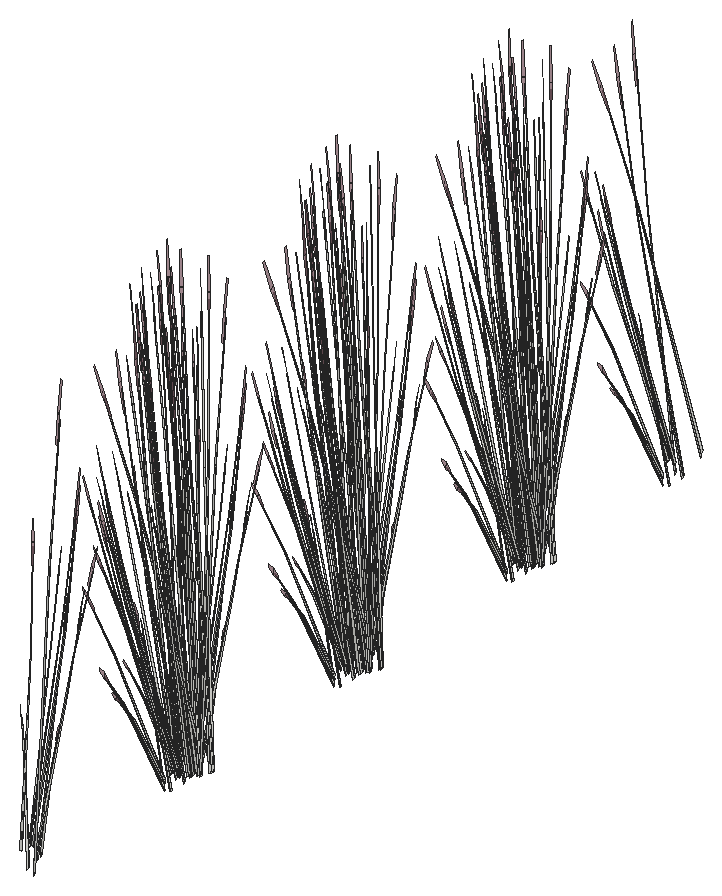
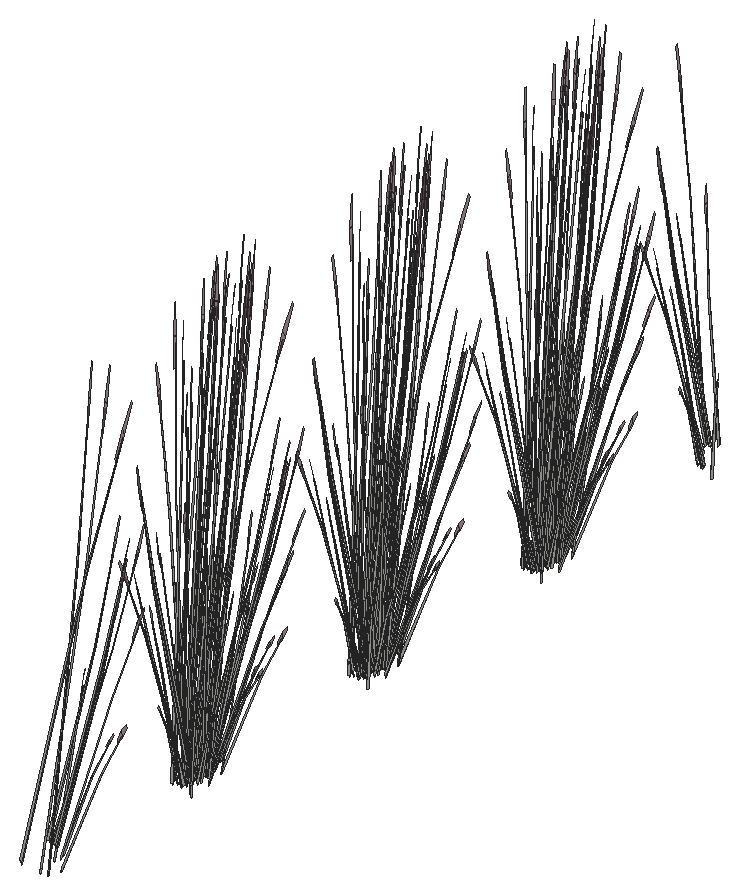
# SketchUp Ruby script. Lengths in inches.
U = 1.inch
M = Sketchup.active_model
def pt(a) = Geom::Point3d.new(a.map { |v| v * U })
def face(e, loops, mat)
  f = e.add_face(loops[0].map { |a| pt(a) })
  loops[1..].each { |l| e.add_face(l.map { |a| pt(a) }).erase! }
  f.material = f.back_material = mat if mat
  f
end
# faces: each face lists its corners as indices into pts; further lists are holes
def faces(e, pts, list, mat = nil) = list.each { |f| face(e, (f[0].is_a?(Array) ? f : [f]).map { |l| l.map { |i| pts[i] } }, mat) }
# xy, xz, yz: faces in a plane at the given z, y or x. An outline is a flat list of corners, or four numbers for a rectangle; further outlines are holes
def ring(l) = l.size == 4 ? [[l[0], l[1]], [l[2], l[1]], [l[2], l[3]], [l[0], l[3]]] : l.each_slice(2).to_a
def flat(e, list, mat, &to3) = list.each { |f| face(e, (f[0].is_a?(Array) ? f : [f]).map { |l| ring(l).map { |u, v| to3.(u, v) } }, mat) }
def xy(e, z, list, mat = nil) = flat(e, list, mat) { |x, y| [x, y, z] }
def xz(e, y, list, mat = nil) = flat(e, list, mat) { |x, z| [x, y, z] }
def yz(e, x, list, mat = nil) = flat(e, list, mat) { |y, z| [x, y, z] }
def lines(e, pts, list) = list.each { |a, b| e.add_line(pt(pts[a]), pt(pts[b])) }
# prism: a flat outline (further loops are holes) pulled along v
def prism(e, loops, v, mat = nil)
  f = face(e, loops, mat); d = Geom::Vector3d.new(v.map { |x| x * U })
  f.pushpull(f.normal.samedirection?(d) ? d.length : -d.length)
end
def box(e, o, s, mat = nil) = prism(e, [[o, [o[0] + s[0], o[1], o[2]], [o[0] + s[0], o[1] + s[1], o[2]], [o[0], o[1] + s[1], o[2]]]], [0, 0, s[2]], mat)
def at(x, y, z, deg = 0) = Geom::Transformation.translation(pt([x, y, z])) * Geom::Transformation.rotation(ORIGIN, Z_AXIS, deg.degrees)
def axes(o, x, y, z) = Geom::Transformation.new([*x, 0, *y, 0, *z, 0, *pt(o).to_a, 1])
def part(name) = M.definitions.add(name)
# library, detail: a bought-in or finely detailed component or shape, given as its bounding box
def library(name, o, s) = part(name).tap { |d| box(d.entities, o, s) }
def detail(e, o, s) = box(e.add_group.entities, o, s)
def put(e, d, t, mat = nil) = e.add_instance(d, t).tap { |i| i.material = mat if mat }
def group(e, t, mat = nil) = e.add_group.tap { |g| g.transformation = t; g.material = mat if mat }.entities
root = M.entities
M.materials.add("LightPink_Translucent").color = [144, 107, 117]
M.materials["LightPink_Translucent"].alpha = 0.75
c1 = part("blade")
p = [[2.15,0.21,22],[0,0.17,0],[0.09,0.45,0],[2.18,0.31,22],[2.29,0.31,22],[0.38,0.45,0],
  [2.48,0.24,33],[2.49,0.24,33],[2.48,0.22,33]]
faces(c1.entities,p,[[0,1,2,3],[4,5,2,3],[6,3,4,7],[8,0,3,6]])
c2 = part("seeds")
p = [[0.3,-0.1,1.38],[-0.01,-0.03,1.59],[-0.01,-0.03,0.03],[0.14,-0.07,-0.07],[0.29,-0.03,3],[0.15,0.01,3.11]]
faces(c2.entities,p,[[0,1,2,3],[1,0,4,5]],"LightPink_Translucent")
c3 = part("blade with seeds")
put(c3.entities,c1,at(0,0,0))
put(c3.entities,c2,axes([2.4,0.25,30.99],[1.5799,-0.05474,1.17369],[-0.12525,1.92788,0.29478],[-0.07173,-0.02425,1.56792]))
put(root,c3,axes([431.05,69.35,2.03],[0.09666,0.50384,-0.43945],[-0.36608,0.08814,-0.34039],[-0.10491,0.13533,0.84085]))
put(root,c3,axes([433.2,68.33,0.44],[-0.01028,-0.51954,1.21494],[0.46521,0.13467,0.51441],[-0.11003,0.28429,1.14681]))
put(root,c3,axes([430.6,70.64,-0.72],[0.05047,0.05513,1.51654],[0.08558,0.51079,-0.23168],[-0.11187,0.10892,0.25832]))
put(root,c3,axes([431.36,70.35,1.89],[-0.2546,0.29052,-0.30456],[-0.24101,-0.33173,0.39319],[-0.03667,0.16855,0.75234]))
put(root,c3,axes([431.52,71.47,0.38],[-0.00974,-0.3281,0.9878],[0.24334,0.23402,0.72577],[-0.04786,0.15639,0.21757]))
put(root,c3,axes([431.61,70.21,2.3],[0.26937,0.37076,-0.48779],[-0.28456,0.3247,-0.37783],[-0.04099,0.18838,0.93334]))
put(root,c3,axes([431.32,70.76,0.43],[0.34184,-0.09771,0.05596],[0.07859,0.39367,-0.74222],[-0.02167,0.19928,0.6653]))
put(root,c3,axes([431.53,70.04,2.59],[-0.00979,0.51041,-0.6782],[-0.4123,-0.03428,0.08184],[-0.04351,0.21623,0.95938]))
put(root,c3,axes([431.24,71.18,0.23],[0.11874,-0.08705,1.22981],[0.29317,0.26247,-0.26449],[-0.08726,0.22711,0.52581]))
put(root,c3,axes([431.39,70.76,0.89],[0.00827,-0.28486,1.32737],[0.37184,0.15046,0.18343],[-0.03222,0.30359,0.62678]))
put(root,c3,axes([432.74,89.46,2.28],[-0.17959,-0.44867,-0.61099],[0.36969,-0.25004,0.07373],[-0.042,-0.21679,0.8643]))
put(root,c3,axes([431.57,88.86,0.23],[-0.02279,0.18051,1.22981],[-0.33311,0.15111,-0.26449],[-0.07787,-0.23331,0.52581]))
put(root,c3,axes([432.6,89.37,2.03],[-0.3699,-0.13833,-0.43945],[0.12679,-0.47426,-0.34039],[-0.03392,-0.19095,0.84085]))
put(root,c3,axes([431.45,88.57,0.38],[0.19628,0.19205,0.9878],[-0.28586,0.11545,0.72577],[-0.06116,-0.1476,0.21757]))
put(root,c3,axes([431.93,89.59,2.28],[-0.32086,-0.26671,-0.61099],[0.22803,-0.46737,0.07373],[-0.11625,-0.15925,0.8643]))
put(root,c3,axes([431.82,89.24,1.89],[-0.05812,-0.44446,-0.30456],[0.33222,-0.11736,0.39319],[-0.08923,-0.12737,0.75234]))
put(root,c3,axes([431.3,89.15,-0.72],[-0.03645,0.07269,1.51654],[-0.36835,0.15672,-0.23168],[-0.08898,-0.14257,0.25832]))
put(root,c3,axes([431.9,91.15,-0.2],[-0.15453,-0.56584,-0.60058],[0.44514,-0.20379,-0.15763],[-0.01708,-0.19161,1.32568]))
put(root,c3,axes([431.78,89.6,2.03],[-0.37131,0.13117,-0.43945],[-0.06495,-0.49674,-0.34039],[-0.09973,-0.14235,0.84085]))
put(root,c3,axes([432.36,88.85,-0.17],[-0.26003,0.31656,-0.03348],[-0.23826,-0.3467,-0.15179],[-0.01677,-0.09824,0.50065]))
put(root,c3,axes([432.69,92.61,0.86],[0.32517,0.22251,1.30084],[-0.31856,0.47936,0.51441],[-0.14269,-0.28411,1.09053]))
put(root,c3,axes([430.99,91.07,-0.26],[0,-0.5518,-0.427],[0.42099,0,0],[0,-0.12568,1.35453]))
put(root,c3,axes([431.05,90.02,1.89],[-0.2141,-0.34548,-0.30456],[0.24447,-0.32704,0.39319],[-0.12421,-0.04976,0.75234]))
put(root,c3,axes([431.17,91.08,-0.26],[0.26266,-0.34428,-0.26641],[0.26266,0.34428,0.26641],[0,-0.11089,1.19518]))
put(root,c3,axes([431.07,89.43,-0.17],[-0.10855,0.45057,-0.03348],[-0.33409,-0.1386,-0.15179],[-0.05073,-0.0737,0.50065]))
put(root,c3,axes([432.09,91.71,0.29],[-0.42377,-0.26329,-0.25022],[0.20405,-0.55571,-0.43002],[-0.01332,-0.13644,1.37348]))
put(root,c3,axes([430.89,91.49,0.04],[-0.47052,0,0],[0,-0.61671,-0.44382],[0,-0.14046,1.40792]))
put(root,c3,axes([430.97,90.38,0.23],[0.07347,0.15363,1.22981],[-0.16929,0.41759,-0.26449],[-0.17383,-0.09981,0.52581]))
put(root,c3,axes([431.27,90.25,2.28],[-0.37615,-0.01329,-0.61099],[0.02526,-0.55946,0.07373],[-0.15935,-0.05904,0.8643]))
put(root,c3,axes([431.25,91.32,0],[-0.35001,0.46392,0.2645],[-0.35022,-0.45904,-0.31383],[-0.01222,-0.13174,1.41801]))
put(root,c3,axes([432.2,92.29,0.1],[0.09973,-0.65385,-0.20149],[0.47288,0.11397,0.44093],[-0.08263,-0.0903,1.34539]))
put(root,c3,axes([431.15,90.36,2.03],[-0.27323,0.36552,-0.43945],[-0.23929,-0.38612,-0.34039],[-0.13882,-0.05561,0.84085]))
put(root,c3,axes([430.53,90.85,0.38],[0.24023,-0.03948,0.9878],[-0.15239,0.3479,0.72577],[-0.11872,-0.05219,0.21757]))
put(root,c3,axes([431.17,91.58,0.13],[0,0.5518,0.427],[-0.42099,0,0],[0,-0.12568,1.35453]))
put(root,c3,axes([432.17,92.03,-0.1],[-0.22605,-0.46315,-0.38476],[0.34239,-0.32614,0.18517],[-0.07315,-0.05731,1.23533]))
put(root,c3,axes([432.13,91.86,0.34],[-0.18257,0.49721,0.38476],[-0.37935,-0.23929,-0.18517],[0,-0.11462,1.23533]))
put(root,c3,axes([431.97,92.2,-0.23],[-0.39143,-0.09047,-0.53624],[0.0826,-0.55804,-0.14074],[-0.11681,-0.06762,1.18365]))
put(root,c3,axes([432.26,91.98,0.03],[0.4756,0.11626,0.39349],[-0.09679,0.6566,0.15441],[-0.0695,-0.0634,1.36617]))
put(root,c3,axes([430.71,91.41,-0.72],[0.00954,0.08696,1.51654],[-0.19238,0.45414,-0.23168],[-0.13665,-0.02289,0.25832]))
put(root,c3,axes([431.55,93.05,-0.26],[-0.08839,-0.48081,-0.26641],[0.35106,-0.13653,0.26641],[-0.07077,-0.05545,1.19518]))
put(root,c3,axes([431.45,93.26,-0.26],[-0.35217,-0.2759,-0.427],[0.2105,-0.49473,0],[-0.08021,-0.06284,1.35453]))
put(root,c3,axes([430.67,91.22,1.89],[-0.31272,-0.15393,-0.30456],[0.09121,-0.44909,0.39319],[-0.1259,0.04118,0.75234]))
put(root,c3,axes([432.41,92.29,0.29],[-0.37992,0.36634,-0.25022],[-0.25264,-0.51764,-0.43002],[-0.09374,-0.05257,1.37348]))
put(root,c3,axes([432.375,92.45,0.25],[-0.07259,0.49245,0.12452],[-0.35466,-0.08548,-0.35559],[-0.06454,-0.05057,1.09]))
put(root,c3,axes([431.62,91.14,0.875],[0.10696,-0.07982,1.52275],[0.03688,0.55733,0.11917],[-0.23167,0.07395,0.54424]))
put(root,c3,axes([432.84,92.45,0.12],[-0.36743,-0.44413,-0.21665],[0.30918,-0.49872,0.47412],[-0.09894,0.05195,1.44665]))
put(root,c3,axes([431.87,93.3,0.13],[0.35217,0.2759,0.427],[-0.2105,0.49473,0],[-0.08021,-0.06284,1.35453]))
put(root,c3,axes([430.88,91.45,2.03],[-0.10194,0.50193,-0.43945],[-0.34951,-0.17204,-0.34039],[-0.14072,0.04602,0.84085]))
put(root,c3,axes([431.67,93.59,0.04],[-0.23526,0.55293,0],[-0.3936,-0.30836,-0.44382],[-0.08964,-0.07023,1.40792]))
put(root,c3,axes([432.65,92.36,-0.1],[-0.40861,0.03406,-0.38476],[-0.03695,-0.56543,0.18517],[-0.07315,0.05731,1.23533]))
put(root,c3,axes([433.1,93.67,-0.11],[-0.23233,-0.55486,-0.04422],[0.3936,-0.30836,0.44382],[-0.09699,0.05283,1.40722]))
put(root,c3,axes([433,93.6,-0.26],[-0.35106,-0.13653,-0.26641],[0.08839,-0.48081,0.26641],[-0.07077,0.05545,1.19518]))
put(root,c3,axes([430.46,92.625,0.23],[0.13077,0.0453,1.22981],[0.08428,0.46268,-0.26449],[-0.17763,0.08661,0.52581]))
put(root,c3,axes([430.19,93.59,0.38],[0.15682,-0.25009,0.9878],[0.06188,0.39591,0.72577],[-0.11333,0.07089,0.21757]))
put(root,c3,axes([432.9375,92.2,0.29],[0.04385,0.62963,-0.25022],[-0.45669,0.03807,-0.43002],[-0.08042,0.08387,1.37348]))
put(root,c3,axes([430.78,92.51,1.89],[-0.32754,0.07886,-0.30456],[-0.08649,-0.45081,0.39319],[-0.09386,0.12109,0.75234]))
put(root,c3,axes([432.66,92.69,-0.23],[-0.25345,0.41475,-0.53624],[-0.31485,-0.37608,-0.14074],[-0.10156,0.10346,1.18365]))
put(root,c3,axes([433.08,93.82,-0.26],[-0.35217,0.2759,-0.427],[-0.2105,-0.49473,0],[-0.08021,0.06284,1.35453]))
put(root,c3,axes([431.05,92.5625,2.03],[0.09666,0.50384,-0.43945],[-0.36608,0.08814,-0.34039],[-0.10491,0.13533,0.84085]))
put(root,c3,axes([433.2,91.54,0.44],[-0.01028,-0.51954,1.21494],[0.46521,0.13467,0.51441],[-0.11003,0.28429,1.14681]))
put(root,c3,axes([430.6,93.85,-0.72],[0.05047,0.05513,1.51654],[0.08558,0.51079,-0.23168],[-0.11187,0.10892,0.25832]))
put(root,c3,axes([431.36,93.56,1.89],[-0.2546,0.29052,-0.30456],[-0.24101,-0.33173,0.39319],[-0.03667,0.16855,0.75234]))
put(root,c3,axes([431.52,94.68,0.38],[-0.00974,-0.3281,0.9878],[0.24334,0.23402,0.72577],[-0.04786,0.15639,0.21757]))
put(root,c3,axes([431.61,93.42,2.3],[0.26937,0.37076,-0.48779],[-0.28456,0.3247,-0.37783],[-0.04099,0.18838,0.93334]))
put(root,c3,axes([431.32,93.97,0.43],[0.34184,-0.09771,0.05596],[0.07859,0.39367,-0.74222],[-0.02167,0.19928,0.6653]))
put(root,c3,axes([431.53,93.25,2.59],[-0.00979,0.51041,-0.6782],[-0.4123,-0.03428,0.08184],[-0.04351,0.21623,0.95938]))
put(root,c3,axes([431.24,94.39,0.23],[0.11874,-0.08705,1.22981],[0.29317,0.26247,-0.26449],[-0.08726,0.22711,0.52581]))
put(root,c3,axes([431.39,93.97,0.89],[0.00827,-0.28486,1.32737],[0.37184,0.15046,0.18343],[-0.03222,0.30359,0.62678]))
put(root,c3,axes([431.57,112.55,0.23],[-0.02279,0.18051,1.22981],[-0.33311,0.15111,-0.26449],[-0.07787,-0.23331,0.52581]))
put(root,c3,axes([432.6,113.06,2.03],[-0.3699,-0.13833,-0.43945],[0.12679,-0.47426,-0.34039],[-0.03392,-0.19095,0.84085]))
put(root,c3,axes([431.45,112.26,0.38],[0.19628,0.19205,0.9878],[-0.28586,0.11545,0.72577],[-0.06116,-0.1476,0.21757]))
put(root,c3,axes([431.93,113.28,2.28],[-0.32086,-0.26671,-0.61099],[0.22803,-0.46737,0.07373],[-0.11625,-0.15925,0.8643]))
put(root,c3,axes([431.82,112.92,1.89],[-0.05812,-0.44446,-0.30456],[0.33222,-0.11736,0.39319],[-0.08923,-0.12737,0.75234]))
put(root,c3,axes([431.3,112.84,-0.72],[-0.03645,0.07269,1.51654],[-0.36835,0.15672,-0.23168],[-0.08898,-0.14257,0.25832]))
put(root,c3,axes([431.9,114.84,-0.2],[-0.15453,-0.56584,-0.60058],[0.44514,-0.20379,-0.15763],[-0.01708,-0.19161,1.32568]))
put(root,c3,axes([431.78,113.29,2.03],[-0.37131,0.13117,-0.43945],[-0.06495,-0.49674,-0.34039],[-0.09973,-0.14235,0.84085]))
put(root,c3,axes([432.36,112.54,-0.17],[-0.26003,0.31656,-0.03348],[-0.23826,-0.3467,-0.15179],[-0.01677,-0.09824,0.50065]))
put(root,c3,axes([432.69,116.29,0.86],[0.32517,0.22251,1.30084],[-0.31856,0.47936,0.51441],[-0.14269,-0.28411,1.09053]))
put(root,c3,axes([430.99,114.76,-0.26],[0,-0.5518,-0.427],[0.42099,0,0],[0,-0.12568,1.35453]))
put(root,c3,axes([431.05,113.71,1.89],[-0.2141,-0.34548,-0.30456],[0.24447,-0.32704,0.39319],[-0.12421,-0.04976,0.75234]))
put(root,c3,axes([431.17,114.77,-0.26],[0.26266,-0.34428,-0.26641],[0.26266,0.34428,0.26641],[0,-0.11089,1.19518]))
put(root,c3,axes([431.07,113.12,-0.17],[-0.10855,0.45057,-0.03348],[-0.33409,-0.1386,-0.15179],[-0.05073,-0.0737,0.50065]))
put(root,c3,axes([432.09,115.39,0.29],[-0.42377,-0.26329,-0.25022],[0.20405,-0.55571,-0.43002],[-0.01332,-0.13644,1.37348]))
put(root,c3,axes([430.89,115.17,0.04],[-0.47052,0,0],[0,-0.61671,-0.44382],[0,-0.14046,1.40792]))
put(root,c3,axes([430.97,114.07,0.23],[0.07347,0.15363,1.22981],[-0.16929,0.41759,-0.26449],[-0.17383,-0.09981,0.52581]))
put(root,c3,axes([431.27,113.9375,2.28],[-0.37615,-0.01329,-0.61099],[0.02526,-0.55946,0.07373],[-0.15935,-0.05904,0.8643]))
put(root,c3,axes([431.25,115.01,0],[-0.35001,0.46392,0.2645],[-0.35022,-0.45904,-0.31383],[-0.01222,-0.13174,1.41801]))
put(root,c3,axes([432.2,115.98,0.1],[0.09973,-0.65385,-0.20149],[0.47288,0.11397,0.44093],[-0.08263,-0.0903,1.34539]))
put(root,c3,axes([431.15,114.05,2.03],[-0.27323,0.36552,-0.43945],[-0.23929,-0.38612,-0.34039],[-0.13882,-0.05561,0.84085]))
put(root,c3,axes([430.53,114.53,0.38],[0.24023,-0.03948,0.9878],[-0.15239,0.3479,0.72577],[-0.11872,-0.05219,0.21757]))
put(root,c3,axes([431.17,115.27,0.13],[0,0.5518,0.427],[-0.42099,0,0],[0,-0.12568,1.35453]))
put(root,c3,axes([432.17,115.71,-0.1],[-0.22605,-0.46315,-0.38476],[0.34239,-0.32614,0.18517],[-0.07315,-0.05731,1.23533]))
put(root,c3,axes([432.13,115.55,0.34],[-0.18257,0.49721,0.38476],[-0.37935,-0.23929,-0.18517],[0,-0.11462,1.23533]))
put(root,c3,axes([431.97,115.89,-0.23],[-0.39143,-0.09047,-0.53624],[0.0826,-0.55804,-0.14074],[-0.11681,-0.06762,1.18365]))
put(root,c3,axes([432.26,115.66,0.03],[0.4756,0.11626,0.39349],[-0.09679,0.6566,0.15441],[-0.0695,-0.0634,1.36617]))
put(root,c3,axes([430.71,115.1,-0.72],[0.00954,0.08696,1.51654],[-0.19238,0.45414,-0.23168],[-0.13665,-0.02289,0.25832]))
put(root,c3,axes([431.55,116.74,-0.26],[-0.08839,-0.48081,-0.26641],[0.35106,-0.13653,0.26641],[-0.07077,-0.05545,1.19518]))
put(root,c3,axes([431.45,116.95,-0.26],[-0.35217,-0.2759,-0.427],[0.2105,-0.49473,0],[-0.08021,-0.06284,1.35453]))
put(root,c3,axes([430.67,114.91,1.89],[-0.31272,-0.15393,-0.30456],[0.09121,-0.44909,0.39319],[-0.1259,0.04118,0.75234]))
put(root,c3,axes([432.41,115.97,0.29],[-0.37992,0.36634,-0.25022],[-0.25264,-0.51764,-0.43002],[-0.09374,-0.05257,1.37348]))
put(root,c3,axes([432.375,116.13,0.25],[-0.07259,0.49245,0.12452],[-0.35466,-0.08548,-0.35559],[-0.06454,-0.05057,1.09]))
put(root,c3,axes([431.62,114.83,0.875],[0.10696,-0.07982,1.52275],[0.03688,0.55733,0.11917],[-0.23167,0.07395,0.54424]))
put(root,c3,axes([432.84,116.14,0.12],[-0.36743,-0.44413,-0.21665],[0.30918,-0.49872,0.47412],[-0.09894,0.05195,1.44665]))
put(root,c3,axes([431.87,116.99,0.13],[0.35217,0.2759,0.427],[-0.2105,0.49473,0],[-0.08021,-0.06284,1.35453]))
put(root,c3,axes([430.88,115.13,2.03],[-0.10194,0.50193,-0.43945],[-0.34951,-0.17204,-0.34039],[-0.14072,0.04602,0.84085]))
put(root,c3,axes([431.67,117.28,0.04],[-0.23526,0.55293,0],[-0.3936,-0.30836,-0.44382],[-0.08964,-0.07023,1.40792]))
put(root,c3,axes([432.65,116.05,-0.1],[-0.40861,0.03406,-0.38476],[-0.03695,-0.56543,0.18517],[-0.07315,0.05731,1.23533]))
put(root,c3,axes([433.1,117.36,-0.11],[-0.23233,-0.55486,-0.04422],[0.3936,-0.30836,0.44382],[-0.09699,0.05283,1.40722]))
put(root,c3,axes([433,117.29,-0.26],[-0.35106,-0.13653,-0.26641],[0.08839,-0.48081,0.26641],[-0.07077,0.05545,1.19518]))
put(root,c3,axes([430.46,116.3125,0.23],[0.13077,0.0453,1.22981],[0.08428,0.46268,-0.26449],[-0.17763,0.08661,0.52581]))
put(root,c3,axes([430.19,117.28,0.38],[0.15682,-0.25009,0.9878],[0.06188,0.39591,0.72577],[-0.11333,0.07089,0.21757]))
put(root,c3,axes([432.9375,115.89,0.29],[0.04385,0.62963,-0.25022],[-0.45669,0.03807,-0.43002],[-0.08042,0.08387,1.37348]))
put(root,c3,axes([430.78,116.2,1.89],[-0.32754,0.07886,-0.30456],[-0.08649,-0.45081,0.39319],[-0.09386,0.12109,0.75234]))
put(root,c3,axes([432.66,116.375,-0.23],[-0.25345,0.41475,-0.53624],[-0.31485,-0.37608,-0.14074],[-0.10156,0.10346,1.18365]))
put(root,c3,axes([433.08,117.51,-0.26],[-0.35217,0.2759,-0.427],[-0.2105,-0.49473,0],[-0.08021,0.06284,1.35453]))
put(root,c3,axes([431.05,116.25,2.03],[0.09666,0.50384,-0.43945],[-0.36608,0.08814,-0.34039],[-0.10491,0.13533,0.84085]))
put(root,c3,axes([433.2,115.23,0.44],[-0.01028,-0.51954,1.21494],[0.46521,0.13467,0.51441],[-0.11003,0.28429,1.14681]))
put(root,c3,axes([430.6,117.54,-0.72],[0.05047,0.05513,1.51654],[0.08558,0.51079,-0.23168],[-0.11187,0.10892,0.25832]))
put(root,c3,axes([431.36,117.24,1.89],[-0.2546,0.29052,-0.30456],[-0.24101,-0.33173,0.39319],[-0.03667,0.16855,0.75234]))
put(root,c3,axes([431.52,118.37,0.38],[-0.00974,-0.3281,0.9878],[0.24334,0.23402,0.72577],[-0.04786,0.15639,0.21757]))
put(root,c3,axes([431.61,117.11,2.3],[0.26937,0.37076,-0.48779],[-0.28456,0.3247,-0.37783],[-0.04099,0.18838,0.93334]))
put(root,c3,axes([431.32,117.66,0.43],[0.34184,-0.09771,0.05596],[0.07859,0.39367,-0.74222],[-0.02167,0.19928,0.6653]))
put(root,c3,axes([431.53,116.9375,2.59],[-0.00979,0.51041,-0.6782],[-0.4123,-0.03428,0.08184],[-0.04351,0.21623,0.95938]))
put(root,c3,axes([431.24,118.08,0.23],[0.11874,-0.08705,1.22981],[0.29317,0.26247,-0.26449],[-0.08726,0.22711,0.52581]))
put(root,c3,axes([431.39,117.66,0.89],[0.00827,-0.28486,1.32737],[0.37184,0.15046,0.18343],[-0.03222,0.30359,0.62678]))
put(root,c3,axes([431.57,136.66,0.23],[-0.02279,0.18051,1.22981],[-0.33311,0.15111,-0.26449],[-0.07787,-0.23331,0.52581]))
put(root,c3,axes([432.6,137.17,2.03],[-0.3699,-0.13833,-0.43945],[0.12679,-0.47426,-0.34039],[-0.03392,-0.19095,0.84085]))
put(root,c3,axes([431.45,136.37,0.38],[0.19628,0.19205,0.9878],[-0.28586,0.11545,0.72577],[-0.06116,-0.1476,0.21757]))
put(root,c3,axes([431.93,137.39,2.28],[-0.32086,-0.26671,-0.61099],[0.22803,-0.46737,0.07373],[-0.11625,-0.15925,0.8643]))
put(root,c3,axes([431.82,137.04,1.89],[-0.05812,-0.44446,-0.30456],[0.33222,-0.11736,0.39319],[-0.08923,-0.12737,0.75234]))
put(root,c3,axes([431.3,136.95,-0.72],[-0.03645,0.07269,1.51654],[-0.36835,0.15672,-0.23168],[-0.08898,-0.14257,0.25832]))
put(root,c3,axes([431.9,138.95,-0.2],[-0.15453,-0.56584,-0.60058],[0.44514,-0.20379,-0.15763],[-0.01708,-0.19161,1.32568]))
put(root,c3,axes([431.78,137.4,2.03],[-0.37131,0.13117,-0.43945],[-0.06495,-0.49674,-0.34039],[-0.09973,-0.14235,0.84085]))
put(root,c3,axes([432.36,136.65,-0.17],[-0.26003,0.31656,-0.03348],[-0.23826,-0.3467,-0.15179],[-0.01677,-0.09824,0.50065]))
put(root,c3,axes([432.69,140.41,0.86],[0.32517,0.22251,1.30084],[-0.31856,0.47936,0.51441],[-0.14269,-0.28411,1.09053]))
put(root,c3,axes([430.99,138.87,-0.26],[0,-0.5518,-0.427],[0.42099,0,0],[0,-0.12568,1.35453]))
put(root,c3,axes([431.05,137.82,1.89],[-0.2141,-0.34548,-0.30456],[0.24447,-0.32704,0.39319],[-0.12421,-0.04976,0.75234]))
put(root,c3,axes([431.17,138.88,-0.26],[0.26266,-0.34428,-0.26641],[0.26266,0.34428,0.26641],[0,-0.11089,1.19518]))
put(root,c3,axes([431.07,137.23,-0.17],[-0.10855,0.45057,-0.03348],[-0.33409,-0.1386,-0.15179],[-0.05073,-0.0737,0.50065]))
put(root,c3,axes([432.09,139.51,0.29],[-0.42377,-0.26329,-0.25022],[0.20405,-0.55571,-0.43002],[-0.01332,-0.13644,1.37348]))
put(root,c3,axes([430.89,139.29,0.04],[-0.47052,0,0],[0,-0.61671,-0.44382],[0,-0.14046,1.40792]))
put(root,c3,axes([430.97,138.18,0.23],[0.07347,0.15363,1.22981],[-0.16929,0.41759,-0.26449],[-0.17383,-0.09981,0.52581]))
put(root,c3,axes([431.27,138.05,2.28],[-0.37615,-0.01329,-0.61099],[0.02526,-0.55946,0.07373],[-0.15935,-0.05904,0.8643]))
put(root,c3,axes([431.25,139.125,0],[-0.35001,0.46392,0.2645],[-0.35022,-0.45904,-0.31383],[-0.01222,-0.13174,1.41801]))
put(root,c3,axes([432.2,140.09,0.1],[0.09973,-0.65385,-0.20149],[0.47288,0.11397,0.44093],[-0.08263,-0.0903,1.34539]))
put(root,c3,axes([431.15,138.16,2.03],[-0.27323,0.36552,-0.43945],[-0.23929,-0.38612,-0.34039],[-0.13882,-0.05561,0.84085]))
put(root,c3,axes([430.53,138.65,0.38],[0.24023,-0.03948,0.9878],[-0.15239,0.3479,0.72577],[-0.11872,-0.05219,0.21757]))
put(root,c3,axes([431.17,139.38,0.13],[0,0.5518,0.427],[-0.42099,0,0],[0,-0.12568,1.35453]))
put(root,c3,axes([432.17,139.82,-0.1],[-0.22605,-0.46315,-0.38476],[0.34239,-0.32614,0.18517],[-0.07315,-0.05731,1.23533]))
put(root,c3,axes([432.13,139.66,0.34],[-0.18257,0.49721,0.38476],[-0.37935,-0.23929,-0.18517],[0,-0.11462,1.23533]))
put(root,c3,axes([431.97,140,-0.23],[-0.39143,-0.09047,-0.53624],[0.0826,-0.55804,-0.14074],[-0.11681,-0.06762,1.18365]))
put(root,c3,axes([432.26,139.78,0.03],[0.4756,0.11626,0.39349],[-0.09679,0.6566,0.15441],[-0.0695,-0.0634,1.36617]))
put(root,c3,axes([430.71,139.21,-0.72],[0.00954,0.08696,1.51654],[-0.19238,0.45414,-0.23168],[-0.13665,-0.02289,0.25832]))
put(root,c3,axes([431.55,140.85,-0.26],[-0.08839,-0.48081,-0.26641],[0.35106,-0.13653,0.26641],[-0.07077,-0.05545,1.19518]))
put(root,c3,axes([431.45,141.06,-0.26],[-0.35217,-0.2759,-0.427],[0.2105,-0.49473,0],[-0.08021,-0.06284,1.35453]))
put(root,c3,axes([430.67,139.02,1.89],[-0.31272,-0.15393,-0.30456],[0.09121,-0.44909,0.39319],[-0.1259,0.04118,0.75234]))
put(root,c3,axes([432.41,140.08,0.29],[-0.37992,0.36634,-0.25022],[-0.25264,-0.51764,-0.43002],[-0.09374,-0.05257,1.37348]))
put(root,c3,axes([432.375,140.24,0.25],[-0.07259,0.49245,0.12452],[-0.35466,-0.08548,-0.35559],[-0.06454,-0.05057,1.09]))
put(root,c3,axes([431.62,138.94,0.875],[0.10696,-0.07982,1.52275],[0.03688,0.55733,0.11917],[-0.23167,0.07395,0.54424]))
put(root,c3,axes([432.84,140.25,0.12],[-0.36743,-0.44413,-0.21665],[0.30918,-0.49872,0.47412],[-0.09894,0.05195,1.44665]))
put(root,c3,axes([431.87,141.1,0.13],[0.35217,0.2759,0.427],[-0.2105,0.49473,0],[-0.08021,-0.06284,1.35453]))
put(root,c3,axes([430.88,139.25,2.03],[-0.10194,0.50193,-0.43945],[-0.34951,-0.17204,-0.34039],[-0.14072,0.04602,0.84085]))
put(root,c3,axes([431.67,141.39,0.04],[-0.23526,0.55293,0],[-0.3936,-0.30836,-0.44382],[-0.08964,-0.07023,1.40792]))
put(root,c3,axes([432.65,140.16,-0.1],[-0.40861,0.03406,-0.38476],[-0.03695,-0.56543,0.18517],[-0.07315,0.05731,1.23533]))
put(root,c3,axes([433.1,141.47,-0.11],[-0.23233,-0.55486,-0.04422],[0.3936,-0.30836,0.44382],[-0.09699,0.05283,1.40722]))
put(root,c3,axes([433,141.4,-0.26],[-0.35106,-0.13653,-0.26641],[0.08839,-0.48081,0.26641],[-0.07077,0.05545,1.19518]))
put(root,c3,axes([430.46,140.42,0.23],[0.13077,0.0453,1.22981],[0.08428,0.46268,-0.26449],[-0.17763,0.08661,0.52581]))
put(root,c3,axes([430.19,141.39,0.38],[0.15682,-0.25009,0.9878],[0.06188,0.39591,0.72577],[-0.11333,0.07089,0.21757]))
put(root,c3,axes([432.9375,140,0.29],[0.04385,0.62963,-0.25022],[-0.45669,0.03807,-0.43002],[-0.08042,0.08387,1.37348]))
put(root,c3,axes([430.78,140.3125,1.89],[-0.32754,0.07886,-0.30456],[-0.08649,-0.45081,0.39319],[-0.09386,0.12109,0.75234]))
put(root,c3,axes([432.66,140.48,-0.23],[-0.25345,0.41475,-0.53624],[-0.31485,-0.37608,-0.14074],[-0.10156,0.10346,1.18365]))
put(root,c3,axes([433.08,141.62,-0.26],[-0.35217,0.2759,-0.427],[-0.2105,-0.49473,0],[-0.08021,0.06284,1.35453]))
put(root,c3,axes([431.05,140.36,2.03],[0.09666,0.50384,-0.43945],[-0.36608,0.08814,-0.34039],[-0.10491,0.13533,0.84085]))
put(root,c3,axes([433.2,139.34,0.44],[-0.01028,-0.51954,1.21494],[0.46521,0.13467,0.51441],[-0.11003,0.28429,1.14681]))
put(root,c3,axes([430.6,141.65,-0.72],[0.05047,0.05513,1.51654],[0.08558,0.51079,-0.23168],[-0.11187,0.10892,0.25832]))
put(root,c3,axes([431.36,141.35,1.89],[-0.2546,0.29052,-0.30456],[-0.24101,-0.33173,0.39319],[-0.03667,0.16855,0.75234]))
put(root,c3,axes([431.52,142.48,0.38],[-0.00974,-0.3281,0.9878],[0.24334,0.23402,0.72577],[-0.04786,0.15639,0.21757]))
put(root,c3,axes([431.61,141.22,2.3],[0.26937,0.37076,-0.48779],[-0.28456,0.3247,-0.37783],[-0.04099,0.18838,0.93334]))
put(root,c3,axes([431.32,141.77,0.43],[0.34184,-0.09771,0.05596],[0.07859,0.39367,-0.74222],[-0.02167,0.19928,0.6653]))
put(root,c3,axes([431.53,141.05,2.59],[-0.00979,0.51041,-0.6782],[-0.4123,-0.03428,0.08184],[-0.04351,0.21623,0.95938]))
put(root,c3,axes([431.24,142.19,0.23],[0.11874,-0.08705,1.22981],[0.29317,0.26247,-0.26449],[-0.08726,0.22711,0.52581]))
put(root,c3,axes([431.39,141.77,0.89],[0.00827,-0.28486,1.32737],[0.37184,0.15046,0.18343],[-0.03222,0.30359,0.62678]))
put(root,c3,axes([431.57,158.51,0.23],[-0.02279,0.18051,1.22981],[-0.33311,0.15111,-0.26449],[-0.07787,-0.23331,0.52581]))
put(root,c3,axes([432.6,159.02,2.03],[-0.3699,-0.13833,-0.43945],[0.12679,-0.47426,-0.34039],[-0.03392,-0.19095,0.84085]))
put(root,c3,axes([431.45,158.22,0.38],[0.19628,0.19205,0.9878],[-0.28586,0.11545,0.72577],[-0.06116,-0.1476,0.21757]))
put(root,c3,axes([431.93,159.24,2.28],[-0.32086,-0.26671,-0.61099],[0.22803,-0.46737,0.07373],[-0.11625,-0.15925,0.8643]))
put(root,c3,axes([431.82,158.89,1.89],[-0.05812,-0.44446,-0.30456],[0.33222,-0.11736,0.39319],[-0.08923,-0.12737,0.75234]))
put(root,c3,axes([431.3,158.8,-0.72],[-0.03645,0.07269,1.51654],[-0.36835,0.15672,-0.23168],[-0.08898,-0.14257,0.25832]))
put(root,c3,axes([431.9,160.8,-0.2],[-0.15453,-0.56584,-0.60058],[0.44514,-0.20379,-0.15763],[-0.01708,-0.19161,1.32568]))
put(root,c3,axes([431.78,159.25,2.03],[-0.37131,0.13117,-0.43945],[-0.06495,-0.49674,-0.34039],[-0.09973,-0.14235,0.84085]))
put(root,c3,axes([432.36,158.5,-0.17],[-0.26003,0.31656,-0.03348],[-0.23826,-0.3467,-0.15179],[-0.01677,-0.09824,0.50065]))
put(root,c3,axes([432.69,162.26,0.86],[0.32517,0.22251,1.30084],[-0.31856,0.47936,0.51441],[-0.14269,-0.28411,1.09053]))
put(root,c3,axes([430.99,160.72,-0.26],[0,-0.5518,-0.427],[0.42099,0,0],[0,-0.12568,1.35453]))
put(root,c3,axes([431.05,159.67,1.89],[-0.2141,-0.34548,-0.30456],[0.24447,-0.32704,0.39319],[-0.12421,-0.04976,0.75234]))
